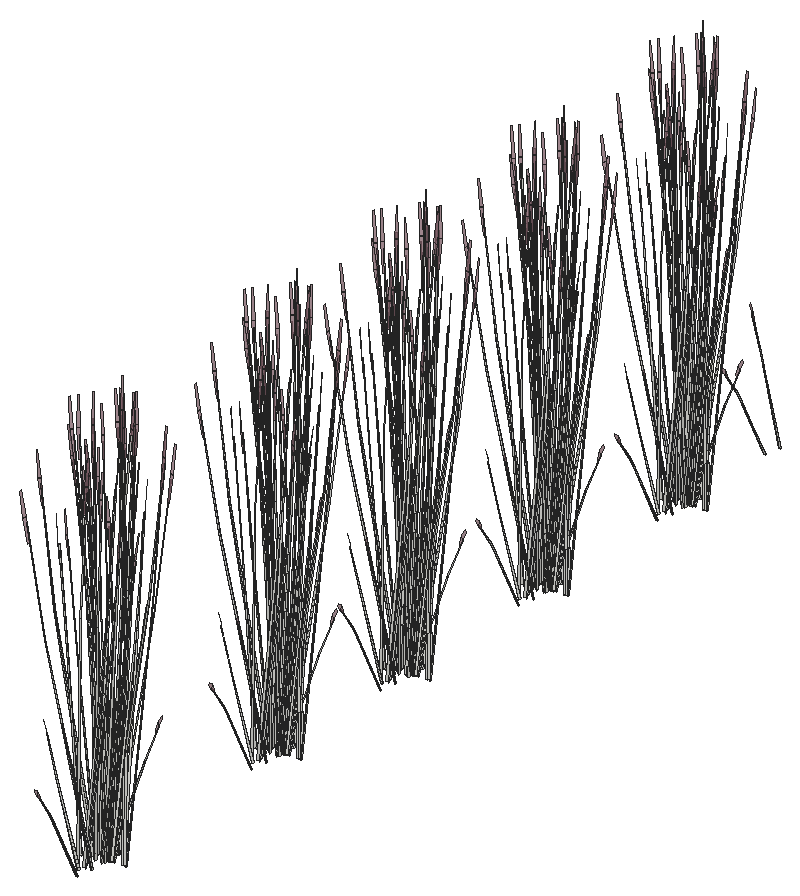
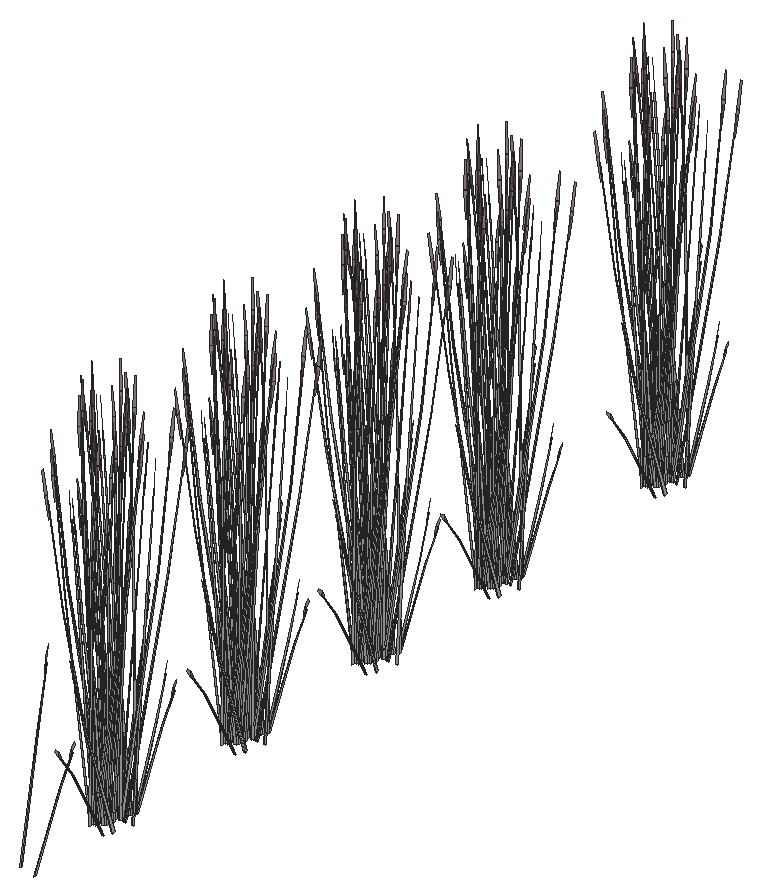
# SketchUp Ruby script. Lengths in inches.
U = 1.inch
M = Sketchup.active_model
def pt(a) = Geom::Point3d.new(a.map { |v| v * U })
def face(e, loops, mat)
  f = e.add_face(loops[0].map { |a| pt(a) })
  loops[1..].each { |l| e.add_face(l.map { |a| pt(a) }).erase! }
  f.material = f.back_material = mat if mat
  f
end
# faces: each face lists its corners as indices into pts; further lists are holes
def faces(e, pts, list, mat = nil) = list.each { |f| face(e, (f[0].is_a?(Array) ? f : [f]).map { |l| l.map { |i| pts[i] } }, mat) }
# xy, xz, yz: faces in a plane at the given z, y or x. An outline is a flat list of corners, or four numbers for a rectangle; further outlines are holes
def ring(l) = l.size == 4 ? [[l[0], l[1]], [l[2], l[1]], [l[2], l[3]], [l[0], l[3]]] : l.each_slice(2).to_a
def flat(e, list, mat, &to3) = list.each { |f| face(e, (f[0].is_a?(Array) ? f : [f]).map { |l| ring(l).map { |u, v| to3.(u, v) } }, mat) }
def xy(e, z, list, mat = nil) = flat(e, list, mat) { |x, y| [x, y, z] }
def xz(e, y, list, mat = nil) = flat(e, list, mat) { |x, z| [x, y, z] }
def yz(e, x, list, mat = nil) = flat(e, list, mat) { |y, z| [x, y, z] }
def lines(e, pts, list) = list.each { |a, b| e.add_line(pt(pts[a]), pt(pts[b])) }
# prism: a flat outline (further loops are holes) pulled along v
def prism(e, loops, v, mat = nil)
  f = face(e, loops, mat); d = Geom::Vector3d.new(v.map { |x| x * U })
  f.pushpull(f.normal.samedirection?(d) ? d.length : -d.length)
end
def box(e, o, s, mat = nil) = prism(e, [[o, [o[0] + s[0], o[1], o[2]], [o[0] + s[0], o[1] + s[1], o[2]], [o[0], o[1] + s[1], o[2]]]], [0, 0, s[2]], mat)
def at(x, y, z, deg = 0) = Geom::Transformation.translation(pt([x, y, z])) * Geom::Transformation.rotation(ORIGIN, Z_AXIS, deg.degrees)
def axes(o, x, y, z) = Geom::Transformation.new([*x, 0, *y, 0, *z, 0, *pt(o).to_a, 1])
def part(name) = M.definitions.add(name)
# library, detail: a bought-in or finely detailed component or shape, given as its bounding box
def library(name, o, s) = part(name).tap { |d| box(d.entities, o, s) }
def detail(e, o, s) = box(e.add_group.entities, o, s)
def put(e, d, t, mat = nil) = e.add_instance(d, t).tap { |i| i.material = mat if mat }
def group(e, t, mat = nil) = e.add_group.tap { |g| g.transformation = t; g.material = mat if mat }.entities
root = M.entities
M.materials.add("LightPink_Translucent").color = [144, 107, 117]
M.materials["LightPink_Translucent"].alpha = 0.75
c1 = part("blade")
p = [[2.15,0.21,22],[0,0.17,0],[0.09,0.45,0],[2.18,0.31,22],[2.29,0.31,22],[0.38,0.45,0],
  [2.48,0.24,33],[2.49,0.24,33],[2.48,0.22,33]]
faces(c1.entities,p,[[0,1,2,3],[4,5,2,3],[6,3,4,7],[8,0,3,6]])
c2 = part("seeds")
p = [[0.3,-0.1,1.38],[-0.01,-0.03,1.59],[-0.01,-0.03,0.03],[0.14,-0.07,-0.07],[0.29,-0.03,3],[0.15,0.01,3.11]]
faces(c2.entities,p,[[0,1,2,3],[1,0,4,5]],"LightPink_Translucent")
c3 = part("blade with seeds")
put(c3.entities,c1,at(0,0,0))
put(c3.entities,c2,axes([2.4,0.25,30.99],[1.5799,-0.05474,1.17369],[-0.12525,1.92788,0.29478],[-0.07173,-0.02425,1.56792]))
put(root,c3,axes([672.94,166.05,512.15],[-0.18493,0.11557,1.18691],[-0.55384,-0.20228,-0.25526],[0.10266,-0.25157,0.50747]))
put(root,c3,axes([671.5625,165.43,511.24],[-0.10912,0.02057,1.46364],[-0.60346,-0.23156,-0.2236],[0.01013,-0.19315,0.24931]))
put(root,c3,axes([670.66,168.2,511.74],[-0.26718,-0.5855,-0.57963],[0.76964,-0.21087,-0.15213],[-0.02953,-0.19827,1.27944]))
put(root,c3,axes([670.56,166.52,511.97],[-0.40676,-0.57214,0],[0.68052,-0.31907,-0.42834],[0.15499,-0.07267,1.3588]))
put(root,c3,axes([671.45,165.83,511.77],[-0.44958,0.32756,-0.03231],[-0.41194,-0.35875,-0.14649],[-0.029,-0.10165,0.48318]))
put(root,c3,axes([671.11,166.43,511.67],[0.60889,-0.28548,-0.4121],[0.36394,0.51192,0],[0.13868,-0.06502,1.30728]))
put(root,c3,axes([671.07,168.35,511.83],[0.31565,-0.51449,-0.37133],[0.65588,0.24761,0.17871],[0,-0.1186,1.19224]))
put(root,c3,axes([671.36,168.1,512.21],[-0.07581,-0.65151,-0.24149],[0.7896,-0.03939,-0.41502],[0.13904,-0.08678,1.32557]))
put(root,c3,axes([669.4,168.13,511.68],[0.45414,-0.35624,-0.25712],[0.45414,0.35624,0.25712],[0,-0.11474,1.15348]))
put(root,c3,axes([670.99,168.78,512.21],[-0.73268,-0.27244,-0.24149],[0.35279,-0.57501,-0.41502],[-0.02303,-0.14118,1.32557]))
put(root,c3,axes([671.25,166.65,511.68],[0.60696,0.14127,-0.25712],[-0.15283,0.49751,0.25712],[0.12236,-0.05737,1.15348]))
put(root,c3,axes([671.46,168.61,512.02],[0.73304,0.27674,0.19974],[-0.35279,0.57501,0.41502],[0,-0.13255,1.3325]))
put(root,c3,axes([671.2,168.43,511.96],[0.28286,0.63846,0.37976],[-0.80821,0.22202,0.14902],[0.00988,-0.11732,1.31851]))
put(root,c3,axes([672.22,168.49,511.83],[0,-0.66065,0],[0.81352,0,0],[0,0,1.48949]))
put(root,c3,axes([671.83,168.07,511.96],[-0.53943,0.51816,0.37976],[-0.64086,-0.4574,0.14902],[0.13005,-0.05171,1.31851]))
put(root,c3,axes([672.42,169,511.91],[-0.60515,-0.49144,-0.05089],[0.60552,-0.49174,0],[-0.02113,-0.01716,1.45724]))
put(root,c3,axes([672.33,167.85,512.17],[0.12551,-0.50956,0.12018],[0.6132,0.08845,-0.34318],[0.1116,0.05232,1.05198]))
put(root,c3,axes([671.27,169.06,511.96],[0.82229,0.1203,0.37976],[-0.16734,0.67942,0.14902],[-0.12017,-0.06561,1.31851]))
put(root,c3,axes([672.77,168.63,511.83],[0.72788,0,0],[0,0.59111,0],[0,0,1.48078]))
put(root,c3,axes([672.53,168.33,511.98],[-0.82229,-0.1203,0.40835],[0.16734,-0.67942,0.16024],[0.12017,0.06561,1.41775]))
put(root,c3,axes([671.88,170.01,511.83],[-0.21227,-0.49226,0],[0.60616,-0.17239,0],[0,0,1.28128]))
put(root,c3,axes([672.75,168.89,511.84],[0.45414,0.3688,0],[-0.45414,0.3688,0],[0,0,1.40491]))
put(root,c3,axes([671.73,170.23,511.82],[-0.65588,-0.25634,0],[0.31565,-0.53263,0],[0,0,1.35047]))
put(root,c3,axes([672.625,168.75,511.9],[0,0.66033,-0.04679],[-0.81352,0,0],[0,0.02075,1.48875]))
put(root,c3,axes([673.02,168.57,512.17],[0.60616,-0.16651,0.12018],[0.21227,0.47548,-0.34318],[0,0.10465,1.05198]))
put(root,c3,axes([672.47,170.24,511.83],[0.65588,0.25634,0],[-0.31565,0.53263,0],[0,0,1.45212]))
put(root,c3,axes([672.73,170.81,511.82],[-0.40169,-0.57414,-0.04268],[0.68052,-0.31907,0.42834],[-0.16769,0.05466,1.35813]))
put(root,c3,axes([672.59,169.42,512.17],[0.48065,0.34305,0.12018],[-0.40092,0.38703,-0.34318],[-0.1116,0.05232,1.05198]))
put(root,c3,axes([672.24,170.03,511.9],[0.28286,0.65594,-0.0499],[-0.80821,0.22985,0],[0.00988,0.02291,1.42904]))
put(root,c3,axes([672.55,170.74,511.68],[-0.60696,-0.14127,-0.25712],[0.15283,-0.49751,0.25712],[-0.12236,0.05737,1.15348]))
put(root,c3,axes([674.57,169.17,511.83],[-0.81312,-0.00457,-0.0413],[0,-0.63814,0.41452],[-0.02555,0.14527,1.31432]))
put(root,c3,axes([672.8125,168.61,512.21],[0.73268,0.27244,-0.24149],[-0.35279,0.57501,-0.41502],[0.02303,0.14118,1.32557]))
put(root,c3,axes([674.4,169.26,511.68],[-0.45414,0.35624,-0.25712],[-0.45414,-0.35624,0.25712],[0,0.11474,1.15348]))
put(root,c3,axes([672.45,169.29,512.21],[0.07581,0.65151,-0.24149],[-0.7896,0.03939,-0.41502],[-0.13904,0.08678,1.32557]))
put(root,c3,axes([672.73,169.04,511.83],[-0.31565,0.51449,-0.37133],[-0.65588,-0.24761,0.17871],[0,0.1186,1.19224]))
put(root,c3,axes([672.75,170.51,511.93],[0.81449,0.18558,0.25528],[-0.20377,0.66335,-0.30288],[-0.13481,0.08302,1.36855]))
put(root,c3,axes([674.72,169.27,511.67],[0,0.57097,-0.4121],[-0.72788,0,0],[0,0.13004,1.30728]))
put(root,c3,axes([673.25,170.875,511.97],[0.40676,0.57214,0],[-0.68052,0.31907,-0.42834],[-0.15499,0.07267,1.3588]))
put(root,c3,axes([673.11,169.19,511.74],[0.23855,0.52277,-0.57446],[-0.68718,0.18827,-0.15077],[0.02637,0.17702,1.26801]))
put(root,c3,axes([671.11,171.05,511.24],[0.10529,-0.03107,1.46364],[0.63335,0.17101,-0.2236],[0.01852,0.19274,0.24931]))
put(root,c3,axes([669.65,171.125,512.34],[0.59102,-0.10111,0.05401],[0.13587,0.40735,-0.71633],[-0.03747,0.2062,0.64209]))
put(root,c3,axes([672.94,193.51,512.15],[-0.18493,0.11557,1.18691],[-0.55384,-0.20228,-0.25526],[0.10266,-0.25157,0.50747]))
put(root,c3,axes([671.5625,192.88,511.24],[-0.10912,0.02057,1.46364],[-0.60346,-0.23156,-0.2236],[0.01013,-0.19315,0.24931]))
put(root,c3,axes([670.66,195.66,511.74],[-0.26718,-0.5855,-0.57963],[0.76964,-0.21087,-0.15213],[-0.02953,-0.19827,1.27944]))
put(root,c3,axes([670.56,193.97,511.97],[-0.40676,-0.57214,0],[0.68052,-0.31907,-0.42834],[0.15499,-0.07267,1.3588]))
put(root,c3,axes([671.45,193.28,511.77],[-0.44958,0.32756,-0.03231],[-0.41194,-0.35875,-0.14649],[-0.029,-0.10165,0.48318]))
put(root,c3,axes([671.11,193.88,511.67],[0.60889,-0.28548,-0.4121],[0.36394,0.51192,0],[0.13868,-0.06502,1.30728]))
put(root,c3,axes([671.07,195.81,511.83],[0.31565,-0.51449,-0.37133],[0.65588,0.24761,0.17871],[0,-0.1186,1.19224]))
put(root,c3,axes([671.36,195.55,512.21],[-0.07581,-0.65151,-0.24149],[0.7896,-0.03939,-0.41502],[0.13904,-0.08678,1.32557]))
put(root,c3,axes([669.4,195.59,511.68],[0.45414,-0.35624,-0.25712],[0.45414,0.35624,0.25712],[0,-0.11474,1.15348]))
put(root,c3,axes([670.99,196.24,512.21],[-0.73268,-0.27244,-0.24149],[0.35279,-0.57501,-0.41502],[-0.02303,-0.14118,1.32557]))
put(root,c3,axes([671.25,194.11,511.68],[0.60696,0.14127,-0.25712],[-0.15283,0.49751,0.25712],[0.12236,-0.05737,1.15348]))
put(root,c3,axes([671.46,196.0625,512.02],[0.73304,0.27674,0.19974],[-0.35279,0.57501,0.41502],[0,-0.13255,1.3325]))
put(root,c3,axes([671.2,195.89,511.96],[0.28286,0.63846,0.37976],[-0.80821,0.22202,0.14902],[0.00988,-0.11732,1.31851]))
put(root,c3,axes([672.22,195.94,511.83],[0,-0.66065,0],[0.81352,0,0],[0,0,1.48949]))
put(root,c3,axes([671.83,195.53,511.96],[-0.53943,0.51816,0.37976],[-0.64086,-0.4574,0.14902],[0.13005,-0.05171,1.31851]))
put(root,c3,axes([672.42,196.45,511.91],[-0.60515,-0.49144,-0.05089],[0.60552,-0.49174,0],[-0.02113,-0.01716,1.45724]))
put(root,c3,axes([672.33,195.3,512.17],[0.12551,-0.50956,0.12018],[0.6132,0.08845,-0.34318],[0.1116,0.05232,1.05198]))
put(root,c3,axes([671.27,196.51,511.96],[0.82229,0.1203,0.37976],[-0.16734,0.67942,0.14902],[-0.12017,-0.06561,1.31851]))
put(root,c3,axes([672.77,196.09,511.83],[0.72788,0,0],[0,0.59111,0],[0,0,1.48078]))
put(root,c3,axes([672.53,195.79,511.98],[-0.82229,-0.1203,0.40835],[0.16734,-0.67942,0.16024],[0.12017,0.06561,1.41775]))
put(root,c3,axes([671.88,197.47,511.83],[-0.21227,-0.49226,0],[0.60616,-0.17239,0],[0,0,1.28128]))
put(root,c3,axes([672.75,196.34,511.84],[0.45414,0.3688,0],[-0.45414,0.3688,0],[0,0,1.40491]))
put(root,c3,axes([671.73,197.69,511.82],[-0.65588,-0.25634,0],[0.31565,-0.53263,0],[0,0,1.35047]))
put(root,c3,axes([672.625,196.21,511.9],[0,0.66033,-0.04679],[-0.81352,0,0],[0,0.02075,1.48875]))
put(root,c3,axes([673.02,196.03,512.17],[0.60616,-0.16651,0.12018],[0.21227,0.47548,-0.34318],[0,0.10465,1.05198]))
put(root,c3,axes([672.47,197.7,511.83],[0.65588,0.25634,0],[-0.31565,0.53263,0],[0,0,1.45212]))
put(root,c3,axes([672.73,198.27,511.82],[-0.40169,-0.57414,-0.04268],[0.68052,-0.31907,0.42834],[-0.16769,0.05466,1.35813]))
put(root,c3,axes([672.59,196.88,512.17],[0.48065,0.34305,0.12018],[-0.40092,0.38703,-0.34318],[-0.1116,0.05232,1.05198]))
put(root,c3,axes([672.24,197.48,511.9],[0.28286,0.65594,-0.0499],[-0.80821,0.22985,0],[0.00988,0.02291,1.42904]))
put(root,c3,axes([672.55,198.19,511.68],[-0.60696,-0.14127,-0.25712],[0.15283,-0.49751,0.25712],[-0.12236,0.05737,1.15348]))
put(root,c3,axes([674.57,196.625,511.83],[-0.81312,-0.00457,-0.0413],[0,-0.63814,0.41452],[-0.02555,0.14527,1.31432]))
put(root,c3,axes([672.8125,196.07,512.21],[0.73268,0.27244,-0.24149],[-0.35279,0.57501,-0.41502],[0.02303,0.14118,1.32557]))
put(root,c3,axes([674.4,196.72,511.68],[-0.45414,0.35624,-0.25712],[-0.45414,-0.35624,0.25712],[0,0.11474,1.15348]))
put(root,c3,axes([672.45,196.75,512.21],[0.07581,0.65151,-0.24149],[-0.7896,0.03939,-0.41502],[-0.13904,0.08678,1.32557]))
put(root,c3,axes([672.73,196.5,511.83],[-0.31565,0.51449,-0.37133],[-0.65588,-0.24761,0.17871],[0,0.1186,1.19224]))
put(root,c3,axes([672.75,197.97,511.93],[0.81449,0.18558,0.25528],[-0.20377,0.66335,-0.30288],[-0.13481,0.08302,1.36855]))
put(root,c3,axes([674.72,196.73,511.67],[0,0.57097,-0.4121],[-0.72788,0,0],[0,0.13004,1.30728]))
put(root,c3,axes([673.25,198.33,511.97],[0.40676,0.57214,0],[-0.68052,0.31907,-0.42834],[-0.15499,0.07267,1.3588]))
put(root,c3,axes([673.11,196.65,511.74],[0.23855,0.52277,-0.57446],[-0.68718,0.18827,-0.15077],[0.02637,0.17702,1.26801]))
put(root,c3,axes([671.11,198.51,511.24],[0.10529,-0.03107,1.46364],[0.63335,0.17101,-0.2236],[0.01852,0.19274,0.24931]))
put(root,c3,axes([669.65,198.58,512.34],[0.59102,-0.10111,0.05401],[0.13587,0.40735,-0.71633],[-0.03747,0.2062,0.64209]))
put(root,c3,axes([672.94,213.8,512.15],[-0.18493,0.11557,1.18691],[-0.55384,-0.20228,-0.25526],[0.10266,-0.25157,0.50747]))
put(root,c3,axes([671.5625,213.17,511.24],[-0.10912,0.02057,1.46364],[-0.60346,-0.23156,-0.2236],[0.01013,-0.19315,0.24931]))
put(root,c3,axes([670.66,215.95,511.74],[-0.26718,-0.5855,-0.57963],[0.76964,-0.21087,-0.15213],[-0.02953,-0.19827,1.27944]))
put(root,c3,axes([670.56,214.27,511.97],[-0.40676,-0.57214,0],[0.68052,-0.31907,-0.42834],[0.15499,-0.07267,1.3588]))
put(root,c3,axes([671.45,213.58,511.77],[-0.44958,0.32756,-0.03231],[-0.41194,-0.35875,-0.14649],[-0.029,-0.10165,0.48318]))
put(root,c3,axes([671.11,214.18,511.67],[0.60889,-0.28548,-0.4121],[0.36394,0.51192,0],[0.13868,-0.06502,1.30728]))
put(root,c3,axes([671.07,216.1,511.83],[0.31565,-0.51449,-0.37133],[0.65588,0.24761,0.17871],[0,-0.1186,1.19224]))
put(root,c3,axes([671.36,215.84,512.21],[-0.07581,-0.65151,-0.24149],[0.7896,-0.03939,-0.41502],[0.13904,-0.08678,1.32557]))
put(root,c3,axes([669.4,215.88,511.68],[0.45414,-0.35624,-0.25712],[0.45414,0.35624,0.25712],[0,-0.11474,1.15348]))
put(root,c3,axes([670.99,216.53,512.21],[-0.73268,-0.27244,-0.24149],[0.35279,-0.57501,-0.41502],[-0.02303,-0.14118,1.32557]))
put(root,c3,axes([671.25,214.4,511.68],[0.60696,0.14127,-0.25712],[-0.15283,0.49751,0.25712],[0.12236,-0.05737,1.15348]))
put(root,c3,axes([671.46,216.36,512.02],[0.73304,0.27674,0.19974],[-0.35279,0.57501,0.41502],[0,-0.13255,1.3325]))
put(root,c3,axes([671.2,216.18,511.96],[0.28286,0.63846,0.37976],[-0.80821,0.22202,0.14902],[0.00988,-0.11732,1.31851]))
put(root,c3,axes([672.22,216.23,511.83],[0,-0.66065,0],[0.81352,0,0],[0,0,1.48949]))
put(root,c3,axes([671.83,215.82,511.96],[-0.53943,0.51816,0.37976],[-0.64086,-0.4574,0.14902],[0.13005,-0.05171,1.31851]))
put(root,c3,axes([672.42,216.75,511.91],[-0.60515,-0.49144,-0.05089],[0.60552,-0.49174,0],[-0.02113,-0.01716,1.45724]))
put(root,c3,axes([671.27,216.81,511.96],[0.82229,0.1203,0.37976],[-0.16734,0.67942,0.14902],[-0.12017,-0.06561,1.31851]))
put(root,c3,axes([672.77,216.38,511.83],[0.72788,0,0],[0,0.59111,0],[0,0,1.48078]))
put(root,c3,axes([672.53,216.08,511.98],[-0.82229,-0.1203,0.40835],[0.16734,-0.67942,0.16024],[0.12017,0.06561,1.41775]))
put(root,c3,axes([671.88,217.76,511.83],[-0.21227,-0.49226,0],[0.60616,-0.17239,0],[0,0,1.28128]))
put(root,c3,axes([672.75,216.64,511.84],[0.45414,0.3688,0],[-0.45414,0.3688,0],[0,0,1.40491]))
put(root,c3,axes([671.73,217.98,511.82],[-0.65588,-0.25634,0],[0.31565,-0.53263,0],[0,0,1.35047]))
put(root,c3,axes([672.625,216.5,511.9],[0,0.66033,-0.04679],[-0.81352,0,0],[0,0.02075,1.48875]))
put(root,c3,axes([673.02,216.32,512.17],[0.60616,-0.16651,0.12018],[0.21227,0.47548,-0.34318],[0,0.10465,1.05198]))
put(root,c3,axes([672.47,217.99,511.83],[0.65588,0.25634,0],[-0.31565,0.53263,0],[0,0,1.45212]))
put(root,c3,axes([672.73,218.56,511.82],[-0.40169,-0.57414,-0.04268],[0.68052,-0.31907,0.42834],[-0.16769,0.05466,1.35813]))
put(root,c3,axes([672.59,217.17,512.17],[0.48065,0.34305,0.12018],[-0.40092,0.38703,-0.34318],[-0.1116,0.05232,1.05198]))
put(root,c3,axes([672.24,217.78,511.9],[0.28286,0.65594,-0.0499],[-0.80821,0.22985,0],[0.00988,0.02291,1.42904]))
put(root,c3,axes([672.55,218.49,511.68],[-0.60696,-0.14127,-0.25712],[0.15283,-0.49751,0.25712],[-0.12236,0.05737,1.15348]))
put(root,c3,axes([674.57,216.92,511.83],[-0.81312,-0.00457,-0.0413],[0,-0.63814,0.41452],[-0.02555,0.14527,1.31432]))
put(root,c3,axes([672.8125,216.36,512.21],[0.73268,0.27244,-0.24149],[-0.35279,0.57501,-0.41502],[0.02303,0.14118,1.32557]))
put(root,c3,axes([674.4,217.01,511.68],[-0.45414,0.35624,-0.25712],[-0.45414,-0.35624,0.25712],[0,0.11474,1.15348]))
put(root,c3,axes([672.45,217.04,512.21],[0.07581,0.65151,-0.24149],[-0.7896,0.03939,-0.41502],[-0.13904,0.08678,1.32557]))
put(root,c3,axes([672.73,216.79,511.83],[-0.31565,0.51449,-0.37133],[-0.65588,-0.24761,0.17871],[0,0.1186,1.19224]))
put(root,c3,axes([672.75,218.26,511.93],[0.81449,0.18558,0.25528],[-0.20377,0.66335,-0.30288],[-0.13481,0.08302,1.36855]))
put(root,c3,axes([674.72,217.02,511.67],[0,0.57097,-0.4121],[-0.72788,0,0],[0,0.13004,1.30728]))
put(root,c3,axes([673.25,218.625,511.97],[0.40676,0.57214,0],[-0.68052,0.31907,-0.42834],[-0.15499,0.07267,1.3588]))
put(root,c3,axes([673.11,216.94,511.74],[0.23855,0.52277,-0.57446],[-0.68718,0.18827,-0.15077],[0.02637,0.17702,1.26801]))
put(root,c3,axes([671.11,218.8,511.24],[0.10529,-0.03107,1.46364],[0.63335,0.17101,-0.2236],[0.01852,0.19274,0.24931]))
put(root,c3,axes([669.65,218.875,512.34],[0.59102,-0.10111,0.05401],[0.13587,0.40735,-0.71633],[-0.03747,0.2062,0.64209]))
put(root,c3,axes([672.94,235.5,512.15],[-0.18493,0.11557,1.18691],[-0.55384,-0.20228,-0.25526],[0.10266,-0.25157,0.50747]))
put(root,c3,axes([671.5625,234.87,511.24],[-0.10912,0.02057,1.46364],[-0.60346,-0.23156,-0.2236],[0.01013,-0.19315,0.24931]))
put(root,c3,axes([670.66,237.65,511.74],[-0.26718,-0.5855,-0.57963],[0.76964,-0.21087,-0.15213],[-0.02953,-0.19827,1.27944]))
put(root,c3,axes([670.56,235.96,511.97],[-0.40676,-0.57214,0],[0.68052,-0.31907,-0.42834],[0.15499,-0.07267,1.3588]))
put(root,c3,axes([671.45,235.27,511.77],[-0.44958,0.32756,-0.03231],[-0.41194,-0.35875,-0.14649],[-0.029,-0.10165,0.48318]))
put(root,c3,axes([671.11,235.875,511.67],[0.60889,-0.28548,-0.4121],[0.36394,0.51192,0],[0.13868,-0.06502,1.30728]))
put(root,c3,axes([671.07,237.8,511.83],[0.31565,-0.51449,-0.37133],[0.65588,0.24761,0.17871],[0,-0.1186,1.19224]))
put(root,c3,axes([671.36,237.54,512.21],[-0.07581,-0.65151,-0.24149],[0.7896,-0.03939,-0.41502],[0.13904,-0.08678,1.32557]))
put(root,c3,axes([669.4,237.58,511.68],[0.45414,-0.35624,-0.25712],[0.45414,0.35624,0.25712],[0,-0.11474,1.15348]))
put(root,c3,axes([670.99,238.22,512.21],[-0.73268,-0.27244,-0.24149],[0.35279,-0.57501,-0.41502],[-0.02303,-0.14118,1.32557]))
put(root,c3,axes([671.25,236.1,511.68],[0.60696,0.14127,-0.25712],[-0.15283,0.49751,0.25712],[0.12236,-0.05737,1.15348]))
put(root,c3,axes([671.46,238.05,512.02],[0.73304,0.27674,0.19974],[-0.35279,0.57501,0.41502],[0,-0.13255,1.3325]))
put(root,c3,axes([671.2,237.88,511.96],[0.28286,0.63846,0.37976],[-0.80821,0.22202,0.14902],[0.00988,-0.11732,1.31851]))
put(root,c3,axes([672.22,237.93,511.83],[0,-0.66065,0],[0.81352,0,0],[0,0,1.48949]))
put(root,c3,axes([671.83,237.52,511.96],[-0.53943,0.51816,0.37976],[-0.64086,-0.4574,0.14902],[0.13005,-0.05171,1.31851]))
put(root,c3,axes([672.42,238.44,511.91],[-0.60515,-0.49144,-0.05089],[0.60552,-0.49174,0],[-0.02113,-0.01716,1.45724]))
put(root,c3,axes([672.33,237.29,512.17],[0.12551,-0.50956,0.12018],[0.6132,0.08845,-0.34318],[0.1116,0.05232,1.05198]))
put(root,c3,axes([671.27,238.5,511.96],[0.82229,0.1203,0.37976],[-0.16734,0.67942,0.14902],[-0.12017,-0.06561,1.31851]))
put(root,c3,axes([672.77,238.08,511.83],[0.72788,0,0],[0,0.59111,0],[0,0,1.48078]))
put(root,c3,axes([672.53,237.78,511.98],[-0.82229,-0.1203,0.40835],[0.16734,-0.67942,0.16024],[0.12017,0.06561,1.41775]))
put(root,c3,axes([671.88,239.46,511.83],[-0.21227,-0.49226,0],[0.60616,-0.17239,0],[0,0,1.28128]))
put(root,c3,axes([672.75,238.33,511.84],[0.45414,0.3688,0],[-0.45414,0.3688,0],[0,0,1.40491]))
put(root,c3,axes([671.73,239.68,511.82],[-0.65588,-0.25634,0],[0.31565,-0.53263,0],[0,0,1.35047]))
put(root,c3,axes([672.625,238.2,511.9],[0,0.66033,-0.04679],[-0.81352,0,0],[0,0.02075,1.48875]))
put(root,c3,axes([673.02,238.02,512.17],[0.60616,-0.16651,0.12018],[0.21227,0.47548,-0.34318],[0,0.10465,1.05198]))
put(root,c3,axes([672.47,239.6875,511.83],[0.65588,0.25634,0],[-0.31565,0.53263,0],[0,0,1.45212]))
put(root,c3,axes([672.73,240.26,511.82],[-0.40169,-0.57414,-0.04268],[0.68052,-0.31907,0.42834],[-0.16769,0.05466,1.35813]))
put(root,c3,axes([672.59,238.87,512.17],[0.48065,0.34305,0.12018],[-0.40092,0.38703,-0.34318],[-0.1116,0.05232,1.05198]))
put(root,c3,axes([672.24,239.47,511.9],[0.28286,0.65594,-0.0499],[-0.80821,0.22985,0],[0.00988,0.02291,1.42904]))
put(root,c3,axes([672.55,240.18,511.68],[-0.60696,-0.14127,-0.25712],[0.15283,-0.49751,0.25712],[-0.12236,0.05737,1.15348]))
put(root,c3,axes([674.57,238.61,511.83],[-0.81312,-0.00457,-0.0413],[0,-0.63814,0.41452],[-0.02555,0.14527,1.31432]))
put(root,c3,axes([672.8125,238.06,512.21],[0.73268,0.27244,-0.24149],[-0.35279,0.57501,-0.41502],[0.02303,0.14118,1.32557]))
put(root,c3,axes([674.4,238.71,511.68],[-0.45414,0.35624,-0.25712],[-0.45414,-0.35624,0.25712],[0,0.11474,1.15348]))
put(root,c3,axes([672.45,238.74,512.21],[0.07581,0.65151,-0.24149],[-0.7896,0.03939,-0.41502],[-0.13904,0.08678,1.32557]))
put(root,c3,axes([672.73,238.49,511.83],[-0.31565,0.51449,-0.37133],[-0.65588,-0.24761,0.17871],[0,0.1186,1.19224]))
put(root,c3,axes([672.75,239.96,511.93],[0.81449,0.18558,0.25528],[-0.20377,0.66335,-0.30288],[-0.13481,0.08302,1.36855]))
put(root,c3,axes([674.72,238.72,511.67],[0,0.57097,-0.4121],[-0.72788,0,0],[0,0.13004,1.30728]))
put(root,c3,axes([673.25,240.32,511.97],[0.40676,0.57214,0],[-0.68052,0.31907,-0.42834],[-0.15499,0.07267,1.3588]))
put(root,c3,axes([673.11,238.64,511.74],[0.23855,0.52277,-0.57446],[-0.68718,0.18827,-0.15077],[0.02637,0.17702,1.26801]))
put(root,c3,axes([671.11,240.49,511.24],[0.10529,-0.03107,1.46364],[0.63335,0.17101,-0.2236],[0.01852,0.19274,0.24931]))
put(root,c3,axes([669.65,240.57,512.34],[0.59102,-0.10111,0.05401],[0.13587,0.40735,-0.71633],[-0.03747,0.2062,0.64209]))
put(root,c3,axes([672.94,257.34,512.15],[-0.18493,0.11557,1.18691],[-0.55384,-0.20228,-0.25526],[0.10266,-0.25157,0.50747]))
put(root,c3,axes([671.5625,256.72,511.24],[-0.10912,0.02057,1.46364],[-0.60346,-0.23156,-0.2236],[0.01013,-0.19315,0.24931]))
put(root,c3,axes([670.66,259.49,511.74],[-0.26718,-0.5855,-0.57963],[0.76964,-0.21087,-0.15213],[-0.02953,-0.19827,1.27944]))
put(root,c3,axes([670.56,257.81,511.97],[-0.40676,-0.57214,0],[0.68052,-0.31907,-0.42834],[0.15499,-0.07267,1.3588]))
put(root,c3,axes([671.45,257.12,511.77],[-0.44958,0.32756,-0.03231],[-0.41194,-0.35875,-0.14649],[-0.029,-0.10165,0.48318]))
put(root,c3,axes([671.11,257.72,511.67],[0.60889,-0.28548,-0.4121],[0.36394,0.51192,0],[0.13868,-0.06502,1.30728]))
put(root,c3,axes([671.07,259.64,511.83],[0.31565,-0.51449,-0.37133],[0.65588,0.24761,0.17871],[0,-0.1186,1.19224]))
put(root,c3,axes([671.36,259.39,512.21],[-0.07581,-0.65151,-0.24149],[0.7896,-0.03939,-0.41502],[0.13904,-0.08678,1.32557]))
put(root,c3,axes([669.4,259.42,511.68],[0.45414,-0.35624,-0.25712],[0.45414,0.35624,0.25712],[0,-0.11474,1.15348]))
put(root,c3,axes([670.99,260.07,512.21],[-0.73268,-0.27244,-0.24149],[0.35279,-0.57501,-0.41502],[-0.02303,-0.14118,1.32557]))
put(root,c3,axes([671.25,257.94,511.68],[0.60696,0.14127,-0.25712],[-0.15283,0.49751,0.25712],[0.12236,-0.05737,1.15348]))
put(root,c3,axes([671.46,259.9,512.02],[0.73304,0.27674,0.19974],[-0.35279,0.57501,0.41502],[0,-0.13255,1.3325]))
put(root,c3,axes([671.2,259.72,511.96],[0.28286,0.63846,0.37976],[-0.80821,0.22202,0.14902],[0.00988,-0.11732,1.31851]))
put(root,c3,axes([672.22,259.78,511.83],[0,-0.66065,0],[0.81352,0,0],[0,0,1.48949]))
put(root,c3,axes([671.83,259.36,511.96],[-0.53943,0.51816,0.37976],[-0.64086,-0.4574,0.14902],[0.13005,-0.05171,1.31851]))
put(root,c3,axes([672.42,260.29,511.91],[-0.60515,-0.49144,-0.05089],[0.60552,-0.49174,0],[-0.02113,-0.01716,1.45724]))
put(root,c3,axes([672.33,259.14,512.17],[0.12551,-0.50956,0.12018],[0.6132,0.08845,-0.34318],[0.1116,0.05232,1.05198]))
put(root,c3,axes([671.27,260.35,511.96],[0.82229,0.1203,0.37976],[-0.16734,0.67942,0.14902],[-0.12017,-0.06561,1.31851]))
put(root,c3,axes([672.77,259.92,511.83],[0.72788,0,0],[0,0.59111,0],[0,0,1.48078]))
put(root,c3,axes([672.53,259.625,511.98],[-0.82229,-0.1203,0.40835],[0.16734,-0.67942,0.16024],[0.12017,0.06561,1.41775]))
put(root,c3,axes([671.88,261.3,511.83],[-0.21227,-0.49226,0],[0.60616,-0.17239,0],[0,0,1.28128]))
put(root,c3,axes([672.75,260.18,511.84],[0.45414,0.3688,0],[-0.45414,0.3688,0],[0,0,1.40491]))
put(root,c3,axes([671.73,261.52,511.82],[-0.65588,-0.25634,0],[0.31565,-0.53263,0],[0,0,1.35047]))
put(root,c3,axes([672.625,260.04,511.9],[0,0.66033,-0.04679],[-0.81352,0,0],[0,0.02075,1.48875]))
put(root,c3,axes([673.02,259.86,512.17],[0.60616,-0.16651,0.12018],[0.21227,0.47548,-0.34318],[0,0.10465,1.05198]))
put(root,c3,axes([672.47,261.53,511.83],[0.65588,0.25634,0],[-0.31565,0.53263,0],[0,0,1.45212]))
put(root,c3,axes([672.73,262.1,511.82],[-0.40169,-0.57414,-0.04268],[0.68052,-0.31907,0.42834],[-0.16769,0.05466,1.35813]))
put(root,c3,axes([672.59,260.71,512.17],[0.48065,0.34305,0.12018],[-0.40092,0.38703,-0.34318],[-0.1116,0.05232,1.05198]))
put(root,c3,axes([672.24,261.32,511.9],[0.28286,0.65594,-0.0499],[-0.80821,0.22985,0],[0.00988,0.02291,1.42904]))
put(root,c3,axes([672.55,262.03,511.68],[-0.60696,-0.14127,-0.25712],[0.15283,-0.49751,0.25712],[-0.12236,0.05737,1.15348]))
put(root,c3,axes([674.57,260.46,511.83],[-0.81312,-0.00457,-0.0413],[0,-0.63814,0.41452],[-0.02555,0.14527,1.31432]))
put(root,c3,axes([672.8125,259.9,512.21],[0.73268,0.27244,-0.24149],[-0.35279,0.57501,-0.41502],[0.02303,0.14118,1.32557]))
put(root,c3,axes([674.4,260.55,511.68],[-0.45414,0.35624,-0.25712],[-0.45414,-0.35624,0.25712],[0,0.11474,1.15348]))
put(root,c3,axes([672.45,260.59,512.21],[0.07581,0.65151,-0.24149],[-0.7896,0.03939,-0.41502],[-0.13904,0.08678,1.32557]))
put(root,c3,axes([672.73,260.33,511.83],[-0.31565,0.51449,-0.37133],[-0.65588,-0.24761,0.17871],[0,0.1186,1.19224]))
put(root,c3,axes([672.75,261.81,511.93],[0.81449,0.18558,0.25528],[-0.20377,0.66335,-0.30288],[-0.13481,0.08302,1.36855]))
put(root,c3,axes([674.72,260.5625,511.67],[0,0.57097,-0.4121],[-0.72788,0,0],[0,0.13004,1.30728]))
put(root,c3,axes([673.25,262.17,511.97],[0.40676,0.57214,0],[-0.68052,0.31907,-0.42834],[-0.15499,0.07267,1.3588]))
put(root,c3,axes([673.11,260.49,511.74],[0.23855,0.52277,-0.57446],[-0.68718,0.18827,-0.15077],[0.02637,0.17702,1.26801]))
put(root,c3,axes([671.11,262.34,511.24],[0.10529,-0.03107,1.46364],[0.63335,0.17101,-0.2236],[0.01852,0.19274,0.24931]))
put(root,c3,axes([669.65,262.42,512.34],[0.59102,-0.10111,0.05401],[0.13587,0.40735,-0.71633],[-0.03747,0.2062,0.64209]))
put(root,c3,axes([672.94,274.2,512.15],[-0.18493,0.11557,1.18691],[-0.55384,-0.20228,-0.25526],[0.10266,-0.25157,0.50747]))
put(root,c3,axes([671.5625,273.58,511.24],[-0.10912,0.02057,1.46364],[-0.60346,-0.23156,-0.2236],[0.01013,-0.19315,0.24931]))
